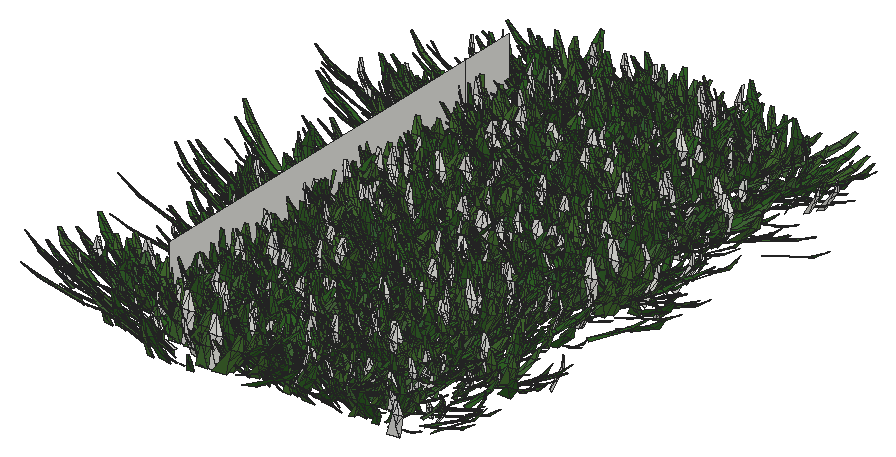
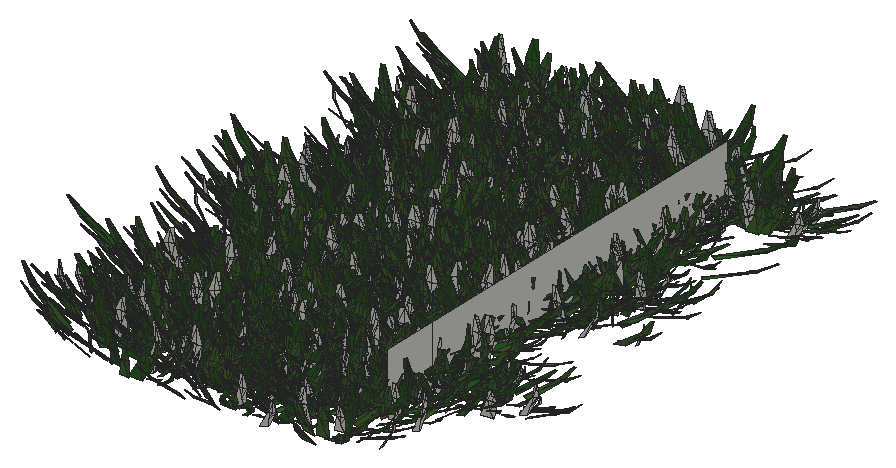
# SketchUp Ruby script. Lengths in inches.
U = 1.inch
M = Sketchup.active_model
def pt(a) = Geom::Point3d.new(a.map { |v| v * U })
def face(e, loops, mat)
  f = e.add_face(loops[0].map { |a| pt(a) })
  loops[1..].each { |l| e.add_face(l.map { |a| pt(a) }).erase! }
  f.material = f.back_material = mat if mat
  f
end
# faces: each face lists its corners as indices into pts; further lists are holes
def faces(e, pts, list, mat = nil) = list.each { |f| face(e, (f[0].is_a?(Array) ? f : [f]).map { |l| l.map { |i| pts[i] } }, mat) }
# xy, xz, yz: faces in a plane at the given z, y or x. An outline is a flat list of corners, or four numbers for a rectangle; further outlines are holes
def ring(l) = l.size == 4 ? [[l[0], l[1]], [l[2], l[1]], [l[2], l[3]], [l[0], l[3]]] : l.each_slice(2).to_a
def flat(e, list, mat, &to3) = list.each { |f| face(e, (f[0].is_a?(Array) ? f : [f]).map { |l| ring(l).map { |u, v| to3.(u, v) } }, mat) }
def xy(e, z, list, mat = nil) = flat(e, list, mat) { |x, y| [x, y, z] }
def xz(e, y, list, mat = nil) = flat(e, list, mat) { |x, z| [x, y, z] }
def yz(e, x, list, mat = nil) = flat(e, list, mat) { |y, z| [x, y, z] }
def lines(e, pts, list) = list.each { |a, b| e.add_line(pt(pts[a]), pt(pts[b])) }
# prism: a flat outline (further loops are holes) pulled along v
def prism(e, loops, v, mat = nil)
  f = face(e, loops, mat); d = Geom::Vector3d.new(v.map { |x| x * U })
  f.pushpull(f.normal.samedirection?(d) ? d.length : -d.length)
end
def box(e, o, s, mat = nil) = prism(e, [[o, [o[0] + s[0], o[1], o[2]], [o[0] + s[0], o[1] + s[1], o[2]], [o[0], o[1] + s[1], o[2]]]], [0, 0, s[2]], mat)
def at(x, y, z, deg = 0) = Geom::Transformation.translation(pt([x, y, z])) * Geom::Transformation.rotation(ORIGIN, Z_AXIS, deg.degrees)
def axes(o, x, y, z) = Geom::Transformation.new([*x, 0, *y, 0, *z, 0, *pt(o).to_a, 1])
def part(name) = M.definitions.add(name)
# library, detail: a bought-in or finely detailed component or shape, given as its bounding box
def library(name, o, s) = part(name).tap { |d| box(d.entities, o, s) }
def detail(e, o, s) = box(e.add_group.entities, o, s)
def put(e, d, t, mat = nil) = e.add_instance(d, t).tap { |i| i.material = mat if mat }
def group(e, t, mat = nil) = e.add_group.tap { |g| g.transformation = t; g.material = mat if mat }.entities
root = M.entities
M.materials.add("Material82").color = [68, 110, 58]
M.materials.add("Material83").color = [48, 90, 38]
M.materials.add("Material84").color = [68, 110, 48]
M.materials.add("Material85").color = [48, 90, 48]
M.materials.add("Material86").color = [58, 110, 58]
M.materials.add("Material87").color = [58, 90, 38]
M.materials.add("Material88").color = [68, 100, 58]
M.materials.add("Material89").color = [48, 100, 38]
c1 = part("grass00")
p = [[-0.6875,0.15,0],[-0.56,0.08,5.52],[-0.04,0.03,2.76],[0.48,-0.02,0],[0.35,-0.02,5.52],[-0.1,-0.14,5.52],
  [-0.12,0.65,8.37],[-0.42,0.65,8.37]]
faces(c1.entities,p,[[0,1,2,3],[3,2,4],[1,5,2],[5,4,2],[1,6,5],[4,5,6],[7,6,1]])
c2 = part("Group16\#1")
put(c2.entities,c1,axes([1.44,-0.61,-0.01],[0.05352,0.12609,0],[-0.10704,0.04543,0.07239],[0.06664,-0.02828,0.11628]),"Material85")
put(c2.entities,c1,axes([0.76,-0.15,-0.01],[0.04676,0.24062,0],[-0.23162,0.04501,0.06642],[0.0652,-0.01267,0.23595]),"Material82")
put(c2.entities,c1,axes([0.79,0.01,-0.01],[-0.00606,0.34651,0],[-0.34381,-0.00602,0.0432],[0.04319,0.00076,0.34386]))
put(c2.entities,c1,axes([1,0.23,-0.01],[-0.07192,0.31144,0],[-0.28722,-0.06632,0.1236],[0.12043,0.02781,0.29478]),"Material84")
put(c2.entities,c1,axes([1.66,0.77,-0.01],[-0.13828,0.29651,0],[-0.21551,-0.1005,0.22471],[0.20365,0.09498,0.23779]),"Material89")
put(c2.entities,c1,axes([0.6875,0.52,-0.01],[-0.18126,0.24051,0],[-0.22746,-0.17142,0.09788],[0.07817,0.05891,0.28481]),"Material84")
put(c2.entities,c1,axes([0.68,0.78,-0.01],[-0.215,0.18688,0],[-0.12385,-0.14248,0.21334],[0.13995,0.16101,0.18878]),"Material82")
put(c2.entities,c1,axes([0.56,1,-0.01],[-0.13756,0.07624,0],[-0.06159,-0.11112,0.0927],[0.04494,0.08108,0.12705]),"Material84")
put(c2.entities,c1,axes([0.2,0.64,-0.01],[-0.23729,0.07254,0],[-0.05711,-0.18681,0.153],[0.04473,0.14632,0.19535]),"Material89")
put(c2.entities,c1,axes([0.0625,0.72,-0.01],[-0.28874,0.02525,0],[-0.02179,-0.24916,0.14647],[0.01276,0.14591,0.25012]),"Material82")
put(c2.entities,c1,axes([-0.08,0.62,-0.01],[-0.34089,-0.04187,0],[0.03255,-0.26504,0.216],[-0.02633,0.21439,0.26703]),"Material89")
put(c2.entities,c1,axes([-0.34,0.98,-0.01],[-0.14314,-0.0493,0],[0.04397,-0.12769,0.06843],[-0.02228,0.0647,0.13505]),"Material89")
put(c2.entities,c1,axes([-0.87,1.45,-0.01],[-0.23488,-0.14114,0],[0.13761,-0.22901,0.06087],[-0.03135,0.05217,0.26717]))
put(c2.entities,c1,axes([-0.72,0.77,-0.01],[-0.14208,-0.13251,0],[0.07209,-0.0773,0.16301],[-0.11118,0.11922,0.1057]),"Material89")
put(c2.entities,c1,axes([-0.62,0.43,-0.01],[-0.14845,-0.21203,0],[0.18654,-0.13061,0.12304],[-0.10079,0.07057,0.22772]),"Material82")
put(c2.entities,c1,axes([-0.68,0.29,-0.01],[-0.13639,-0.32136,0],[0.31723,-0.13464,0.05579],[-0.05136,0.0218,0.34462]),"Material83")
put(c2.entities,c1,axes([-0.64,0.125,-0.01],[-0.0458,-0.23569,0],[0.22124,-0.043,0.08276],[-0.08124,0.01579,0.22538]),"Material86")
put(c2.entities,c1,axes([-1.6,-0.03,-0.01],[0.00576,-0.32897,0],[0.27526,0.00482,0.18018],[-0.18015,-0.00315,0.2753]),"Material84")
put(c2.entities,c1,axes([-1.36,-0.31,-0.01],[0.05718,-0.24765,0],[0.18172,0.04196,0.17267],[-0.16825,-0.03885,0.1865]),"Material89")
put(c2.entities,c1,axes([-1.54,-0.72,-0.01],[0.06537,-0.14017,0],[0.13555,0.06321,0.03939],[-0.0357,-0.01665,0.14956]))
put(c2.entities,c1,axes([-1.19,-0.9,-0.01],[0.09597,-0.12735,0],[0.11214,0.08451,0.07557],[-0.06035,-0.04548,0.14042]),"Material88")
put(c2.entities,c1,axes([-0.47,-0.54,-0.01],[0.11588,-0.10072,0],[0.0618,0.0711,0.12124],[-0.07953,-0.0915,0.0942]))
put(c2.entities,c1,axes([-0.47,-0.84,-0.01],[0.11927,-0.0661,0],[0.06603,0.11913,0.00646],[-0.00313,-0.00565,0.13621]),"Material84")
put(c2.entities,c1,axes([-0.38,-1.24,-0.01],[0.28037,-0.08571,0],[0.0618,0.20215,0.20315],[-0.05939,-0.19428,0.21139]),"Material88")
put(c2.entities,c1,axes([-0.06,-0.66,-0.01],[0.22719,-0.01987,0],[0.01247,0.14255,0.17758],[-0.01547,-0.17691,0.1431]),"Material87")
put(c2.entities,c1,axes([0.11,-0.89,-0.01],[0.14882,0.01828,0],[-0.01058,0.08611,0.12229],[0.01491,-0.12138,0.08676]),"Material85")
put(c2.entities,c1,axes([0.25,-0.72,-0.01],[0.20481,0.07053,0],[-0.06206,0.18022,0.10291],[0.03351,-0.0973,0.1906]),"Material85")
put(c2.entities,c1,axes([0.85,-1.42,-0.01],[0.16481,0.09904,0],[-0.09472,0.15762,0.05616],[0.02893,-0.04814,0.18389]),"Material84")
put(c2.entities,c1,axes([1.01,-1.09,-0.01],[0.21858,0.20385,0],[-0.17495,0.1876,0.15339],[0.10462,-0.11218,0.25652]),"Material89")
put(c2.entities,c1,axes([1.01,-0.71,-0.01],[0.08733,0.12473,0],[-0.06445,0.04512,0.13037],[0.1068,-0.07477,0.07867]),"Material85")
c3 = part("Group15\#1")
put(c3.entities,c2,at(0,0,0))
c4 = part("3darcstudiotree_grass00\#1")
put(c4.entities,c3,at(0,0,0))
yz(root,1674.65,[[1000.12,-29.74,1040.81,-23.22],[1040.81,-29.74,1046.93,-23.22]])
put(root,c4,axes([1682.48,994.64,-29.74],[1.98347,-1.087,0],[3.74124,1.06175,-0.05142],[0.23843,0.06767,1.97373]))
put(root,c4,axes([1688.78,996.4,-29.74],[3.93037,0.00712,0],[-0.01552,1.3324,-0.03904],[-0.00131,0.11261,1.85207]))
put(root,c4,axes([1678.21,996.72,-29.74],[1.61856,-1.20753,0],[3.98562,0.83088,-0.05061],[0.25894,0.05398,1.95538]))
put(root,c4,axes([1693.57,996.73,-29.74],[3.29344,0.56908,0],[-1.86687,1.68036,-0.0492],[-0.08744,0.0787,1.54416]))
put(root,c4,axes([1672.86,997.4,-29.74],[3.81318,-1.10593,0],[2.582,1.38461,-0.02397],[0.05758,0.03088,1.32443]))
put(root,c4,axes([1699.31,996.68,-29.74],[-4.26775,-0.24104,0],[0.59342,-1.63411,-0.00988],[0.00789,-0.02172,1.76639]))
put(root,c4,axes([1684.36,997.08,-29.74],[-2.26608,1.33318,0],[-3.11704,-0.82402,-0.02214],[-0.10686,-0.02825,1.63462]))
put(root,c4,axes([1693.35,998.28,-29.74],[-0.80049,-1.46058,0],[4.26303,-0.36338,-0.06129],[0.24511,-0.02089,1.3376]))
put(root,c4,axes([1698.59,998.75,-29.74],[2.46062,-1.19689,0],[3.08233,0.98555,-0.02965],[0.1062,0.03396,1.3715]))
put(root,c4,axes([1689.9,998.23,-29.74],[0.74688,1.42324,0],[-4.33801,0.35406,-0.00233],[-0.01216,0.00099,1.77271]))
put(root,c4,axes([1684.75,998.98,-29.74],[0.44293,-1.56057,0],[3.90028,0.17217,-0.04376],[0.2246,0.00991,1.51939]))
put(root,c4,axes([1679.33,999.11,-29.74],[-2.26232,-1.46372,0],[3.35674,-0.80691,-0.05337],[0.23381,-0.0562,1.5119]))
put(root,c4,axes([1672.04,999.74,-29.74],[3.91343,0.66663,0],[-1.38696,1.26634,-0.02193],[-0.04877,0.04453,1.47013]))
put(root,c4,axes([1678.79,1000.89,-29.74],[2.08347,-1.59715,0],[3.15506,0.64012,-0.03693],[0.21917,0.04447,1.77491]))
put(root,c4,axes([1671.84,1000.72,-29.74],[-0.96185,1.4826,0],[-3.70839,-0.37418,-0.04208],[-0.21883,-0.02208,1.54007]))
put(root,c4,axes([1701.59,1000.91,-29.74],[-0.04598,1.31401,0],[-3.68449,-0.02005,-0.02407],[-0.13013,-0.00071,1.49365]))
put(root,c4,axes([1682.94,1000.99,-29.74],[-4.22007,0.35003,0],[-0.86715,-1.62599,-0.01674],[-0.0198,-0.03713,1.81501]))
put(root,c4,axes([1690.11,1001.33,-29.74],[-4.17152,-0.5223,0],[1.23744,-1.53711,-0.0262],[0.03523,-0.04376,1.36239]))
put(root,c4,axes([1692.61,1001.72,-29.74],[-4.50934,-0.15911,0],[0.38591,-1.70103,-0.03473],[0.01636,-0.07211,1.7157]))
put(root,c4,axes([1678.41,1002.77,-29.74],[3.33408,0.32893,0],[-1.10916,1.74856,-0.00744],[-0.00738,0.01164,1.4009]))
put(root,c4,axes([1684.8125,1003.25,-29.74],[3.70469,-0.86578,0],[1.68851,1.12372,-0.02001],[0.07058,0.04697,1.71774]))
put(root,c4,axes([1693.88,1003.15,-29.74],[-2.35898,-1.49879,0],[3.37563,-0.82632,-0.02087],[0.09435,-0.0231,1.58468]))
put(root,c4,axes([1690.36,1004.02,-29.74],[3.46997,0.08994,0],[-0.27266,1.63611,-0.01423],[-0.00549,0.03292,1.83161]))
put(root,c4,axes([1698.24,1003.53,-29.74],[-3.51315,0.12017,0],[-0.35069,-1.59447,-0.04163],[-0.0224,-0.10183,1.89396]))
put(root,c4,axes([1698.43,1004.86,-29.74],[-1.97176,-1.44506,0],[3.679,-0.78074,-0.04084],[0.18174,-0.03857,1.58232]))
put(root,c4,axes([1681.61,1005.79,-29.74],[3.27704,0.72692,0],[-1.98468,1.39155,-0.00275],[-0.00611,0.00428,1.37565]))
put(root,c4,axes([1688.03,1005.77,-29.74],[4.00271,0.72936,0],[-1.54017,1.31459,-0.00765],[-0.0159,0.01357,1.36419]))
put(root,c4,axes([1695.67,1006.16,-29.74],[0.6786,-1.83556,0],[4.57598,0.26311,-0.00277],[0.01184,0.00068,1.49508]))
put(root,c4,axes([1677.09,1006.07,-29.74],[-0.56456,1.41966,0],[-3.50259,-0.21664,-0.01794],[-0.10644,-0.00658,1.59592]))
put(root,c4,axes([1699.12,1007.01,-29.74],[-0.79088,1.37944,0],[-4.55872,-0.4065,-0.04071],[-0.16308,-0.01454,1.43871]))
put(root,c4,axes([1689.47,1007.97,-29.74],[-2.17228,-1.46024,0],[3.41853,-0.79094,-0.03431],[0.15337,-0.03548,1.53951]))
put(root,c4,axes([1704.14,1008.1,-29.74],[0.08239,-1.33128,0],[3.65037,0.03514,-0.00377],[0.02295,0.00022,1.66719]))
put(root,c4,axes([1677.83,1007.79,-29.74],[0.79004,1.45858,0],[-4.26548,0.35933,-0.00171],[-0.00893,0.00075,1.74655]))
put(root,c4,axes([1682.12,1007.79,-29.74],[-4.09965,-0.15274,0],[0.36855,-1.53851,-0.03137],[0.01329,-0.05547,1.3228]))
put(root,c4,axes([1693,1008.21,-29.74],[2.33704,1.50763,0],[-2.98263,0.71909,-0.02868],[-0.14145,0.0341,1.51486]))
put(root,c4,axes([1683.55,1009.36,-29.74],[-2.87872,-0.88154,0],[2.80816,-1.42624,-0.06125],[0.14894,-0.07565,1.36064]))
put(root,c4,axes([1676.9,1009.375,-29.74],[-4.49567,-0.3985,0],[0.83225,-1.46029,-0.03373],[0.03467,-0.06083,1.33323]))
put(root,c4,axes([1694.31,1009.95,-29.74],[2.20491,1.1875,0],[-2.92266,0.84401,-0.01948],[-0.09978,0.02881,1.72408]))
put(root,c4,axes([1688.37,1010.37,-29.74],[2.24844,-1.02464,0],[3.26531,1.11441,-0.03846],[0.14191,0.04843,1.57923]))
put(root,c4,axes([1698.08,1010.42,-29.74],[-0.43927,-1.56699,0],[3.3973,-0.14812,-0.00454],[0.02991,-0.0013,1.6986]))
put(root,c4,axes([1698.99,1011.78,-29.74],[3.02682,0.57541,0],[-1.48298,1.21327,-0.04063],[-0.10557,0.08637,1.53169]))
put(root,c4,axes([1676.83,1011.58,-29.74],[-4.6805,0.28538,0],[-0.54089,-1.37973,-0.03554],[-0.03758,-0.09587,1.83631]))
put(root,c4,axes([1684.43,1012.25,-29.74],[-2.16844,-1.41891,0],[2.90956,-0.69156,-0.03107],[0.17396,-0.04135,1.66455]))
put(root,c4,axes([1694.86,1012.31,-29.74],[3.34663,1.11106,0],[-2.8307,1.32609,-0.01247],[-0.04541,0.02127,1.86292]))
put(root,c4,axes([1689.1,1012.13,-29.74],[0.76665,1.71699,0],[-3.34963,0.23261,-0.02162],[-0.1104,0.00767,1.32159]))
put(root,c4,axes([1695.96,1013.62,-29.74],[1.99944,-1.04992,0],[3.08282,0.91308,-0.00267],[0.01382,0.00409,1.87177]))
put(root,c4,axes([1698.68,1013.75,-29.74],[3.2382,0.426,0],[-1.27463,1.50694,-0.00681],[-0.01361,0.01609,1.90695]))
put(root,c4,axes([1676.4,1013.78,-29.74],[-0.79677,-1.6402,0],[3.36468,-0.25421,-0.01579],[0.08769,-0.00662,1.45182]))
put(root,c4,axes([1690.1,1013.5,-29.74],[-3.49855,-0.51529,0],[1.58914,-1.67809,-0.03885],[0.07118,-0.07517,1.78292]))
put(root,c4,axes([1683.1,1014.37,-29.74],[0.11814,-1.8536,0],[3.92163,0.03887,-0.05528],[0.30038,0.00298,1.59813]))
put(root,c4,axes([1682.57,1015.82,-29.74],[-1.51918,-1.57572,0],[4.39344,-0.65879,-0.02869],[0.10716,-0.01607,1.40786]))
put(root,c4,axes([1693.29,1015.89,-29.74],[-1.29023,-1.58759,0],[3.9469,-0.49888,-0.03893],[0.19606,-0.02478,1.64312]))
put(root,c4,axes([1690.52,1016.06,-29.74],[-3.86459,-0.0799,0],[0.17825,-1.34085,-0.00586],[0.00206,-0.0155,1.71352]))
put(root,c4,axes([1676.37,1015.95,-29.74],[-3.29804,1.27107,0],[-2.52678,-1.01968,-0.01484],[-0.07094,-0.02863,1.85373]))
put(root,c4,axes([1672.71,1016.58,-29.74],[3.70183,0.03147,0],[-0.07805,1.42775,-0.0399],[-0.00598,0.10931,1.8861]))
put(root,c4,axes([1700.56,1016.74,-29.74],[3.67827,0.2088,0],[-0.57305,1.57009,-0.04848],[-0.0346,0.09479,1.51023]))
put(root,c4,axes([1675.55,1018.06,-29.74],[-0.10316,1.55622,0],[-4.09748,-0.04224,-0.03889],[-0.19104,-0.00197,1.50954]))
put(root,c4,axes([1673.3,1018.61,-29.74],[-0.3225,-1.34219,0],[4.58247,-0.17125,-0.03587],[0.16603,-0.0062,1.60406]))
put(root,c4,axes([1693.55,1018.6,-29.74],[-3.37238,-1.2695,0],[3.05865,-1.2637,-0.04863],[0.19789,-0.08176,1.95701]))
put(root,c4,axes([1688.3,1019.23,-29.74],[3.40582,0.10745,0],[-0.34866,1.71886,-0.00093],[-0.00031,0.0015,1.35201]))
put(root,c4,axes([1699,1019.08,-29.74],[-1.25158,-1.24653,0],[3.09013,-0.48255,-0.01359],[0.08484,-0.01325,1.67314]))
put(root,c4,axes([1682.28,1019.12,-29.74],[-1.65501,1.23077,0],[-2.99443,-0.62625,-0.02105],[-0.13776,-0.02881,1.88169]))
put(root,c4,axes([1678.88,1020.41,-29.74],[2.10633,-1.56652,0],[4.07545,0.85227,-0.05067],[0.19625,0.04104,1.51576]))
put(root,c4,axes([1697.78,1020.07,-29.74],[-3.55958,-1.14913,0],[2.41323,-1.16263,-0.04086],[0.15936,-0.07677,1.75811]))
put(root,c4,axes([1688.81,1020.68,-29.74],[2.63669,-1.45672,0],[3.66232,1.03098,-0.04124],[0.15536,0.04373,1.56101]))
put(root,c4,axes([1682.3125,1020.17,-29.74],[-1.69964,1.49974,0],[-3.25198,-0.57319,-0.0353],[-0.21623,-0.03811,1.79152]))
put(root,c4,axes([1693.32,1021.25,-29.74],[-3.5162,-0.01544,0],[0.03762,-1.33225,-0.02017],[0.00158,-0.05579,1.77597]))
put(root,c4,axes([1676.5,1022.61,-29.74],[2.48968,-1.1461,0],[2.93182,0.99053,-0.00664],[0.0258,0.00872,1.48048]))
put(root,c4,axes([1688.37,1022.29,-29.74],[-0.28743,1.31478,0],[-4.42266,-0.15037,-0.00545],[-0.03167,-0.00108,1.93955]))
put(root,c4,axes([1672.85,1022.93,-29.74],[3.82293,-1.07301,0],[2.00012,1.10831,-0.02041],[0.08948,0.04958,1.95445]))
put(root,c4,axes([1701.66,1023.46,-29.74],[1.80491,-1.57701,0],[4.14536,0.7379,-0.03311],[0.16907,0.03009,1.9099]))
put(root,c4,axes([1684.46,1023.57,-29.74],[-1.1098,-1.31734,0],[3.29231,-0.43138,-0.00285],[0.02011,-0.00264,1.93438]))
put(root,c4,axes([1695.87,1023.23,-29.74],[-3.77729,0.83126,0],[-1.83032,-1.29355,-0.03544],[-0.09552,-0.06751,1.55733]))
put(root,c4,axes([1689.85,1024.77,-29.74],[0.50947,-1.51274,0],[4.49668,0.23554,-0.03191],[0.15996,0.00838,1.71939]))
put(root,c4,axes([1681.57,1025.21,-29.74],[-3.21191,1.28173,0],[-2.59769,-1.01243,-0.03007],[-0.15402,-0.06003,1.97134]))
put(root,c4,axes([1698.41,1025.53,-29.74],[-2.97894,1.37787,0],[-2.78264,-0.93567,-0.01811],[-0.06538,-0.02199,1.30017]))
put(root,c4,axes([1696.13,1025.7,-29.74],[-3.83744,0.33373,0],[-0.9251,-1.65441,-0.02531],[-0.02998,-0.05361,1.77094]))
put(root,c4,axes([1677.07,1026.02,-29.74],[1.96349,1.64722,0],[-3.56633,0.66117,-0.03464],[-0.18907,0.03505,1.78143]))
put(root,c4,axes([1701.4375,1027.18,-29.74],[1.28722,-1.76401,0],[4.46987,0.50729,-0.04991],[0.26732,0.03034,1.94306]))
put(root,c4,axes([1703.71,1026.63,-29.74],[-1.91663,1.65988,0],[-3.0087,-0.54032,-0.04508],[-0.21948,-0.03942,1.32557]))
put(root,c4,axes([1677.95,1027.125,-29.74],[-1.20508,-1.27416,0],[3.97727,-0.58504,-0.0406],[0.22085,-0.03249,1.84742]))
put(root,c4,axes([1693.29,1027.625,-29.74],[0.71095,-1.43364,0],[4.62721,0.35689,-0.06032],[0.23627,0.01822,1.41053]))
put(root,c4,axes([1689.14,1028.21,-29.74],[-4.16983,-0.88311,0],[1.85574,-1.3628,-0.02099],[0.05036,-0.03698,1.49075]))
put(root,c4,axes([1684.66,1028.125,-29.74],[-3.85239,-0.20163,0],[0.58764,-1.74619,-0.01228],[0.0079,-0.02349,1.63767]))
put(root,c4,axes([1694.18,1028.78,-29.74],[3.70622,-0.07941,0],[0.19617,1.42399,-0.02262],[0.0073,0.05302,1.6131]))
put(root,c4,axes([1689.12,1029.1,-29.74],[-1.93961,-1.1589,0],[2.81158,-0.73187,-0.03406],[0.19491,-0.05074,1.73123]))
put(root,c4,axes([1700.5,1029.82,-29.74],[0.12202,-1.72029,0],[4.34373,0.04792,-0.00421],[0.02346,0.00026,1.81536]))
put(root,c4,axes([1684.71,1029.31,-29.74],[-1.66799,1.12199,0],[-3.57556,-0.82672,-0.01566],[-0.07039,-0.01628,1.61828]))
put(root,c4,axes([1679.55,1030.15,-29.74],[1.69514,-1.26112,0],[3.85825,0.80658,-0.01977],[0.09529,0.01992,1.78562]))
put(root,c4,axes([1694.82,1031.72,-29.74],[-0.8203,-1.58295,0],[4.36315,-0.35165,-0.03636],[0.17472,-0.01408,1.63697]))
put(root,c4,axes([1700.06,1031.5,-29.74],[-4.26886,-0.01451,0],[0.03771,-1.72573,-0.00939],[0.00047,-0.02147,1.9024]))
put(root,c4,axes([1689.19,1031.88,-29.74],[3.91894,1.05311,0],[-2.36552,1.3691,-0.06012],[-0.14517,0.08402,1.3502]))
put(root,c4,axes([1681.53,1032.22,-29.74],[3.33812,-0.00931,0],[0.03014,1.68097,-0.0442],[0.00131,0.07293,1.33678]))
put(root,c4,axes([1679.48,1032.4,-29.74],[-2.43659,-1.39628,0],[3.54139,-0.96116,-0.05298],[0.19991,-0.05426,1.4759]))
put(root,c4,axes([1676.7,1033.15,-29.74],[-3.06856,1.30795,0],[-2.89535,-1.05647,-0.0352],[-0.142,-0.05181,1.62511]))
put(root,c4,axes([1689.125,1033.87,-29.74],[0.60137,-1.69863,0],[3.35822,0.18491,-0.0384],[0.22932,0.01263,1.53253]))
put(root,c4,axes([1681.72,1033.97,-29.74],[-0.2328,1.40639,0],[-3.78045,-0.09733,-0.01044],[-0.05523,-0.00142,1.50484]))
put(root,c4,axes([1697.59,1034.41,-29.74],[-0.96459,1.39728,0],[-4.50708,-0.48391,-0.06593],[-0.29103,-0.03125,1.60187]))
put(root,c4,axes([1695.9375,1034.51,-29.74],[0.06651,1.49398,0],[-4.62108,0.032,-0.00579],[-0.03066,0.00021,1.83497]))
put(root,c4,axes([1692.92,1035.59,-29.74],[3.81628,-0.13918,0],[0.37321,1.59155,-0.00914],[0.00528,0.02252,1.90465]))
put(root,c4,axes([1689.3,1035.87,-29.74],[-1.5249,1.25696,0],[-3.62628,-0.68422,-0.02774],[-0.1175,-0.02217,1.41462]))
put(root,c4,axes([1682.29,1035.92,-29.74],[-1.7842,1.38137,0],[-4.14651,-0.83297,-0.01882],[-0.07173,-0.01441,1.49212]))
put(root,c4,axes([1675.49,1036.78,-29.74],[-1.63198,-1.29559,0],[3.66951,-0.7189,-0.01655],[0.08632,-0.01691,1.78815]))
put(root,c4,axes([1700.12,1036.6,-29.74],[-0.60649,1.78928,0],[-3.60415,-0.19,-0.04319],[-0.29403,-0.0155,1.87209]))
put(root,c4,axes([1688.54,1037.8125,-29.74],[3.33503,1.17525,0],[-2.6851,1.18507,-0.00121],[-0.00399,0.00176,1.48985]))
put(root,c4,axes([1699.57,1038.03,-29.74],[-1.50368,1.17097,0],[-3.52829,-0.70467,-0.03106],[-0.12382,-0.02473,1.32443]))
put(root,c4,axes([1692.97,1038.73,-29.74],[0.14571,-1.35454,0],[4.55175,0.07615,-0.04061],[0.20314,0.0034,1.70991]))
put(root,c4,axes([1671.8,1038.85,-29.74],[2.90846,1.13793,0],[-2.61613,1.03996,-0.02475],[-0.10205,0.04057,1.62992]))
put(root,c4,axes([1675.59,1039,-29.74],[0.65055,1.72425,0],[-3.43127,0.20135,-0.01524],[-0.11013,0.00646,1.90022]))
put(root,c4,axes([1684.26,1039,-29.74],[-2.50108,0.95556,0],[-2.98511,-1.21518,-0.02879],[-0.10959,-0.04461,1.7592]))
put(root,c4,axes([1671.91,1039.85,-29.74],[4.3644,0.14123,0],[-0.27589,1.32601,-0.01884],[-0.00836,0.04017,1.37151]))
put(root,c4,axes([1681.9,1039.84,-29.74],[-0.81871,-1.45227,0],[3.80429,-0.33355,-0.01455],[0.06635,-0.00582,1.36448]))
put(root,c4,axes([1701.5,1040.27,-29.74],[3.40778,-1.13854,0],[2.78991,1.29874,-0.02128],[0.06823,0.03176,1.60475]))
put(root,c4,axes([1679.52,1040.36,-29.74],[1.18703,1.24458,0],[-3.56072,0.52819,-0.04913],[-0.2933,0.04351,1.81865]))
put(root,c4,axes([1687.29,1040.91,-29.74],[4.2261,-0.33522,0],[0.81524,1.59847,-0.02659],[0.0257,0.05039,1.51897]))
put(root,c4,axes([1694.03,1041.3125,-29.74],[-4.64372,0.01964,0],[-0.04703,-1.72937,-0.01941],[-0.00122,-0.04491,1.92834]))
put(root,c4,axes([1684.09,1042.34,-29.74],[0.27542,-1.59187,0],[4.66457,0.12552,-0.02398],[0.0893,0.0024,1.30813]))
put(root,c4,axes([1676.65,1042.02,-29.74],[-3.57616,-1.16474,0],[2.7999,-1.33704,-0.02974],[0.0776,-0.03706,1.35064]))
put(root,c4,axes([1694.01,1042.93,-29.74],[4.39151,-0.30239,0],[0.81207,1.8342,-0.04063],[0.02885,0.06516,1.46079]))
put(root,c4,axes([1687.96,1042.89,-29.74],[0.23544,-1.60034,0],[3.90526,0.08936,-0.02273],[0.11635,0.00266,1.50351]))
put(root,c4,axes([1699.71,1043.24,-29.74],[2.16016,-1.57069,0],[3.42867,0.73339,-0.01711],[0.07383,0.01579,1.43496]))
put(root,c4,axes([1677.14,1044.58,-29.74],[3.96997,0.02835,0],[-0.08063,1.7564,-0.04973],[-0.00512,0.11159,1.89995]))
put(root,c4,axes([1682.49,1044.57,-29.74],[-3.18032,-1.25414,0],[2.9494,-1.16324,-0.05204],[0.20858,-0.08226,1.77215]))
put(root,c4,axes([1688.08,1044.68,-29.74],[3.671,0.98063,0],[-2.61565,1.5229,-0.02464],[-0.07837,0.04563,1.98292]))
put(root,c4,axes([1692.59,1045.12,-29.74],[3.22571,-1.00591,0],[2.69072,1.34198,-0.01988],[0.07446,0.03714,1.96304]))
put(root,c4,axes([1698.96,1045.67,-29.74],[-1.03876,-1.58927,0],[3.98467,-0.40506,-0.01269],[0.06748,-0.00686,1.69312]))
put(root,c4,axes([1676.21,1046.54,-29.74],[2.6716,0.78375,0],[-2.01413,1.06781,-0.0148],[-0.06741,0.03574,1.93047]))
put(root,c4,axes([1681.16,1046.79,-29.74],[-4.17606,0.09309,0],[-0.21865,-1.52546,-0.00256],[-0.00085,-0.00591,1.70382]))
put(root,c4,axes([1686.62,1047.54,-29.74],[-3.25209,-0.85971,0],[2.35344,-1.3846,-0.05337],[0.14871,-0.08749,1.58535]))
put(root,c4,axes([1701.31,1047.75,-29.74],[-2.22741,-1.08823,0],[2.74712,-0.87452,-0.02577],[0.11865,-0.03777,1.56591]))
put(root,c4,axes([1693.64,1047.5,-29.74],[-3.60513,-0.15499,0],[0.46196,-1.67121,-0.01401],[0.00822,-0.02974,1.72979]))
put(root,c4,axes([1701.18,1048.46,-29.74],[-2.63384,-1.55649,0],[3.02127,-0.79514,-0.04802],[0.24921,-0.06559,1.69851]))
put(root,c4,axes([1682.73,1048.55,-29.74],[-0.69591,-1.28996,0],[3.84518,-0.32263,-0.04713],[0.24772,-0.02078,1.58351]))
put(root,c4,axes([1696.0625,1048.65,-29.74],[4.30833,-0.24109,0],[0.6166,1.71371,-0.05794],[0.04515,0.12549,1.82474]))
put(root,c4,axes([1678.87,1049.1,-29.74],[3.37733,-0.03199,0],[0.10215,1.67739,-0.04057],[0.00409,0.06713,1.33829]))
put(root,c4,axes([1687.6875,1049.92,-29.74],[-3.50198,-0.71469,0],[1.86103,-1.41828,-0.02021],[0.05866,-0.0447,1.91641]))
put(root,c4,axes([1700.85,1050.91,-29.74],[2.75838,0.79761,0],[-2.27657,1.22449,-0.01003],[-0.02813,0.01513,1.36834]))
put(root,c4,axes([1693.97,1050.65,-29.74],[-1.99433,1.44629,0],[-3.30766,-0.70937,-0.03157],[-0.17706,-0.03797,1.80167]))
put(root,c4,axes([1689.45,1051.35,-29.74],[3.4743,0.19553,0],[-0.61359,1.69568,-0.03434],[-0.02545,0.07034,1.70799]))
put(root,c4,axes([1683.66,1050.96,-29.74],[-4.09244,0.60833,0],[-1.31907,-1.38013,-0.00238],[-0.00395,-0.00413,1.31717]))
put(root,c4,axes([1677.47,1052.08,-29.74],[1.23256,1.36805,0],[-3.36714,0.47182,-0.0026],[-0.01342,0.00188,1.46428]))
put(root,c4,axes([1687.3,1053.15,-29.74],[2.94498,0.60485,0],[-2.04543,1.54892,-0.0178],[-0.03241,0.02454,1.30843]))
put(root,c4,axes([1698.72,1053.375,-29.74],[-4.3017,0.59676,0],[-1.104,-1.2377,-0.00518],[-0.01285,-0.0144,1.86492]))
